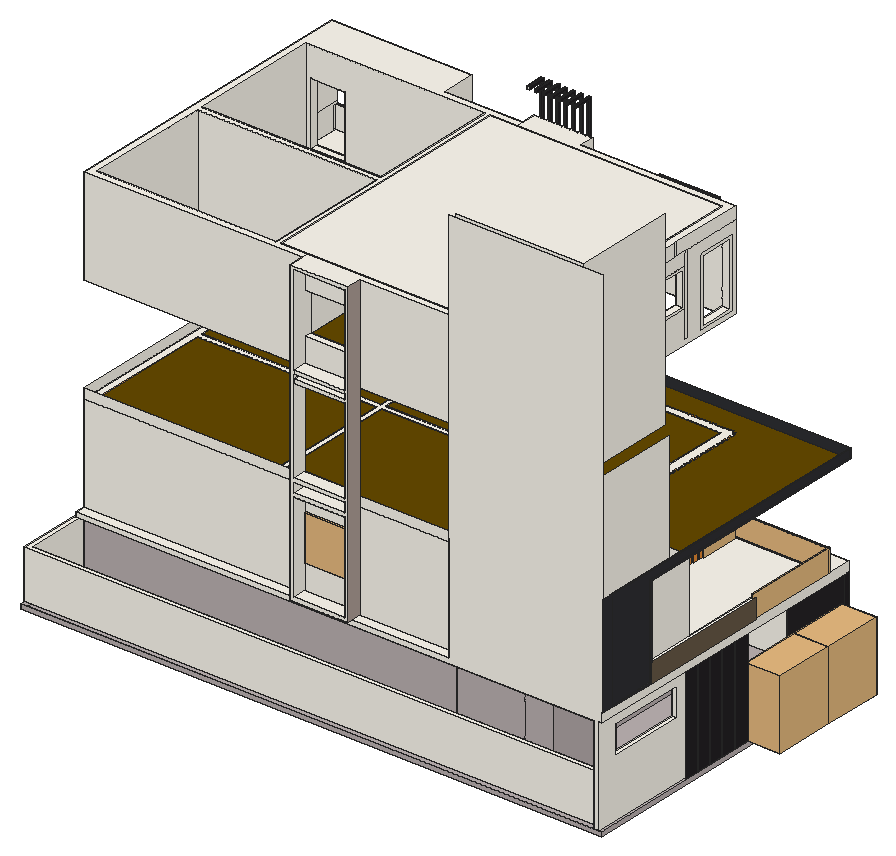
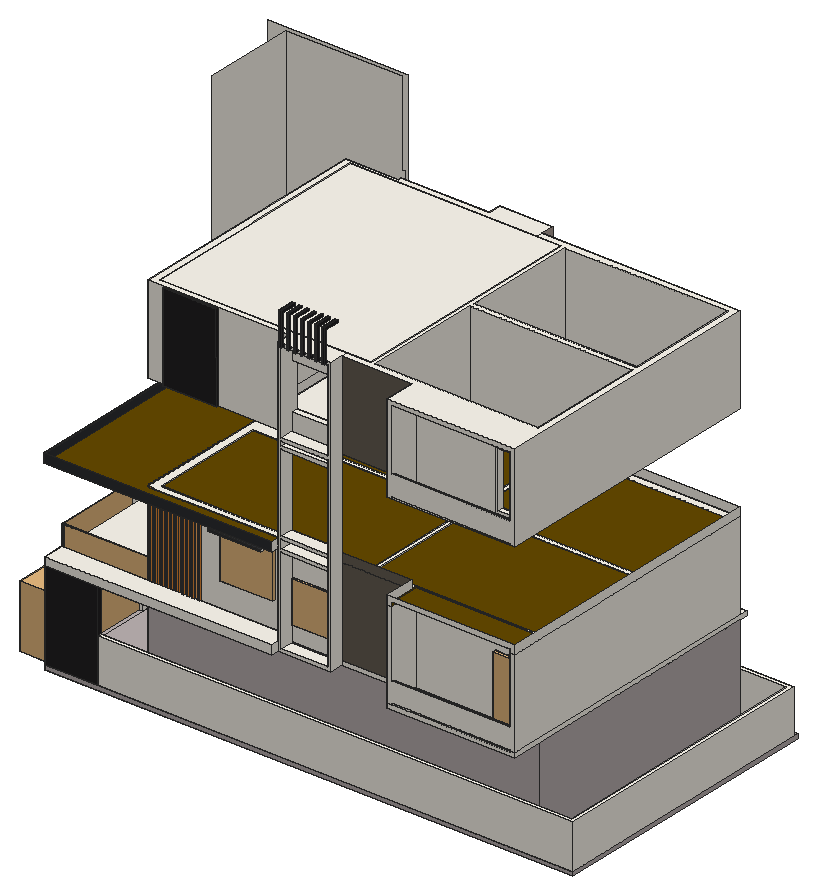
# SketchUp Ruby script. Lengths in inches.
U = 1.inch
M = Sketchup.active_model
def pt(a) = Geom::Point3d.new(a.map { |v| v * U })
def face(e, loops, mat)
  f = e.add_face(loops[0].map { |a| pt(a) })
  loops[1..].each { |l| e.add_face(l.map { |a| pt(a) }).erase! }
  f.material = f.back_material = mat if mat
  f
end
# faces: each face lists its corners as indices into pts; further lists are holes
def faces(e, pts, list, mat = nil) = list.each { |f| face(e, (f[0].is_a?(Array) ? f : [f]).map { |l| l.map { |i| pts[i] } }, mat) }
# xy, xz, yz: faces in a plane at the given z, y or x. An outline is a flat list of corners, or four numbers for a rectangle; further outlines are holes
def ring(l) = l.size == 4 ? [[l[0], l[1]], [l[2], l[1]], [l[2], l[3]], [l[0], l[3]]] : l.each_slice(2).to_a
def flat(e, list, mat, &to3) = list.each { |f| face(e, (f[0].is_a?(Array) ? f : [f]).map { |l| ring(l).map { |u, v| to3.(u, v) } }, mat) }
def xy(e, z, list, mat = nil) = flat(e, list, mat) { |x, y| [x, y, z] }
def xz(e, y, list, mat = nil) = flat(e, list, mat) { |x, z| [x, y, z] }
def yz(e, x, list, mat = nil) = flat(e, list, mat) { |y, z| [x, y, z] }
def lines(e, pts, list) = list.each { |a, b| e.add_line(pt(pts[a]), pt(pts[b])) }
# prism: a flat outline (further loops are holes) pulled along v
def prism(e, loops, v, mat = nil)
  f = face(e, loops, mat); d = Geom::Vector3d.new(v.map { |x| x * U })
  f.pushpull(f.normal.samedirection?(d) ? d.length : -d.length)
end
def box(e, o, s, mat = nil) = prism(e, [[o, [o[0] + s[0], o[1], o[2]], [o[0] + s[0], o[1] + s[1], o[2]], [o[0], o[1] + s[1], o[2]]]], [0, 0, s[2]], mat)
def at(x, y, z, deg = 0) = Geom::Transformation.translation(pt([x, y, z])) * Geom::Transformation.rotation(ORIGIN, Z_AXIS, deg.degrees)
def axes(o, x, y, z) = Geom::Transformation.new([*x, 0, *y, 0, *z, 0, *pt(o).to_a, 1])
def part(name) = M.definitions.add(name)
# library, detail: a bought-in or finely detailed component or shape, given as its bounding box
def library(name, o, s) = part(name).tap { |d| box(d.entities, o, s) }
def detail(e, o, s) = box(e.add_group.entities, o, s)
def put(e, d, t, mat = nil) = e.add_instance(d, t).tap { |i| i.material = mat if mat }
def group(e, t, mat = nil) = e.add_group.tap { |g| g.transformation = t; g.material = mat if mat }.entities
root = M.entities
M.materials.add("B04_Peach_Ember").color = [234, 141, 54]
M.materials.add("C01_Vanilla_Cream").color = [255, 251, 241]
M.materials.add("C03_Honey_Glow").color = [255, 178, 101]
M.materials.add("D08_Bronzed_Mustard").color = [102, 74, 0]
M.materials.add("Forest_Floor_01_1K").color = [106, 91, 72]
M.materials.add("Glass_Basic_1").color = [161, 173, 186]
M.materials["Glass_Basic_1"].alpha = 0.25
M.materials.add("Marble_07_1K").color = [36, 34, 36]
M.materials.add("Plaster_04_1K").color = [106, 98, 87]
M.materials.add("ThomThom - Buttons1").color = [48, 49, 53]
M.materials.add("ThomThom - Complexion1").color = [190, 180, 180]
M.materials.add("ThomThom - Hair1").color = [178, 163, 155]
c1 = library("porta+4",[0.2,-5.42,1.33],[46.55,4.72,83.21])
c2 = library("Ornamental gate leaf",[0,0,0],[161.42,42.43,280.3])
c3 = part("cong")
put(c3.entities,c2,axes([244.78,234.5625,0],[-1,0,0],[0,1,0],[0,0,1]))
put(c3.entities,c2,at(244.78,234.5625,0))
c4 = library("mesh-163",[-551.08,-704.17,-20.03],[1929.24,1401.85,86.96])
c5 = part("Group11")
put(c5.entities,c4,at(0,0,0))
c6 = library("Modern+Gate+1",[0,0,0],[118.11,1.97,78.74])
xy(root,0,[[0,6,720,389.16]],"ThomThom - Complexion1")
xy(root,6,[[711,6,717,138],[648,383.16,720,389.16]],"C01_Vanilla_Cream")
xy(root,6,[[0,6,9,389.16],[[9,6,711,389.16],[69,18,69,360,531,360,531,27,645,27,645,114,651,114,651,18]],[711,6,720,389.16],[78,27,300,183],[306,27,522,183],
  [78,189,300,351],[306,189,522,351]],"ThomThom - Complexion1")
xy(root,78,[[711,30,717,126]],"C01_Vanilla_Cream")
xy(root,114,[[711,30,717,126]],"C01_Vanilla_Cream")
xy(root,126,[[69,6,69,402,243,402,243,360,411,360,411,383.16,720,383.16,720,6,717,6,717,138,711,138,711,6],[411,383.16,648,389.16],[648,383.16,720,389.16]],"C01_Vanilla_Cream")
xy(root,126,[[531,18,651,18,651,114,645,114,645,27,531,27]],"ThomThom - Complexion1")
xy(root,132,[[69,6,531,6,531,190.4375,591.62,190.4375,591.62,348.27,531,348.27,531,360,243,360,243,402,69,402],[531,348.27,603,360]],"C01_Vanilla_Cream")
xy(root,138,[[537,12,693.41,12,693.41,144,718,144,718,241.67,720,241.67,720,357,603,357,603,348.27,591.62,348.27,591.62,190.4375,531,190.4375,531,24,537,24],[603,357,720,360],[411,360,720,389.16]],"C01_Vanilla_Cream")
xy(root,138,[[720,6,722,241.67]],"ThomThom - Buttons1")
xy(root,139,[[720,19,722,80]],"ThomThom - Buttons1")
xy(root,162,[[718,81,722,241.67]],"C01_Vanilla_Cream")
xy(root,252,[[537,12,603,24],[718,81,722,144]],"C01_Vanilla_Cream")
xy(root,252,[[69,18,69,402,75,402,75,360,237,360,237,402,243,402,243,360,411,360,411,389.16,722,389.16,722,144,603,144,603,24,531,24,531,18]],"D08_Bronzed_Mustard")
xy(root,253,[[720,80,722,144],[720,144,722,388.16]],"ThomThom - Buttons1")
xy(root,257.2,[[75,360,237,402]],"D08_Bronzed_Mustard")
xy(root,263,[[720,19,722,144],[720,144,722,388.16]],"ThomThom - Buttons1")
xz(root,6,[[711,6,717,6,717,126,720,126,720,138,722,138,722,624,531,624,531,132,69,132,69,126,711,126]],"C01_Vanilla_Cream")
xz(root,6,[[0,0,720,6]],"ThomThom - Complexion1")
xz(root,12,[[537,138,537,252,603,252,603,264,537,264,537,378,663.55,378,663.55,384,531,384,531,510,535,510,535,624,693.41,624,693.41,138]],"C01_Vanilla_Cream")
xz(root,18,[[69,252,531,264]],"C01_Vanilla_Cream")
xz(root,18,[[531,6,615,126],[615,6,651,126]],"ThomThom - Complexion1")
xz(root,19,[[720,139,722,263]],"ThomThom - Buttons1")
xz(root,24,[[531,138,537,252],[531,252,537,264],[537,252,603,264]],"C01_Vanilla_Cream")
xz(root,27,[[531,6,609,126],[609,6,642.82,126],[642.82,6,645,126]],"ThomThom - Complexion1")
xz(root,30,[[711,78,717,114]],"C01_Vanilla_Cream")
xz(root,80,[[720,139,722,253]],"ThomThom - Buttons1")
xz(root,81,[[718,162,722,252]],"C01_Vanilla_Cream")
xz(root,114,[[645,6,651,126]],"ThomThom - Complexion1")
xz(root,126,[[711,78,717,114]],"C01_Vanilla_Cream")
xz(root,144,[[693.41,138,718,252],[603,252,693.41,264]],"C01_Vanilla_Cream")
xz(root,190.4375,[[531,132,591.62,138]],"C01_Vanilla_Cream")
xz(root,241.67,[[718,138,722,162]],"C01_Vanilla_Cream")
xz(root,348.27,[[591.62,132,603,138]],"C01_Vanilla_Cream")
xz(root,360,[[243,126,411,132],[411,132,603,138]],"C01_Vanilla_Cream")
xz(root,360,[[75,252,237,257.2]],"D08_Bronzed_Mustard")
xz(root,360,[[243,252,411,264]],"Plaster_04_1K")
xz(root,360,[[[347.5,154.65,403.5,210.65],[351.5,158.65,399.5,206.65]]],"ThomThom - Complexion1")
xz(root,383.16,[[648,6,720,126]],"Marble_07_1K")
xz(root,388.16,[[720,253,722,263]],"ThomThom - Buttons1")
xz(root,389.16,[[411,126,720,138]],"C01_Vanilla_Cream")
xz(root,389.16,[[648,6,720,126]],"Marble_07_1K")
xz(root,389.16,[[411,252,722,264]],"ThomThom - Buttons1")
xz(root,389.16,[[0,0,720,6]],"ThomThom - Complexion1")
xz(root,402,[[69,126,243,132],[69,252,69,264,243,264,243,252,237,252,237,257.2,75,257.2,75,252]],"C01_Vanilla_Cream")
yz(root,0,[[6,0,389.16,6]],"ThomThom - Complexion1")
yz(root,69,[[6,126,402,132],[18,252,402,264]],"C01_Vanilla_Cream")
yz(root,75,[[360,252,402,257.2]],"D08_Bronzed_Mustard")
yz(root,237,[[360,252,402,257.2]],"D08_Bronzed_Mustard")
yz(root,243,[[360,126,402,132],[360,252,402,264]],"C01_Vanilla_Cream")
yz(root,411,[[360,126,389.16,138],[360,252,389.16,264]],"C01_Vanilla_Cream")
yz(root,531,[[6,132,6,252,24,252,24,138,190.4375,138,190.4375,132],[6,252,18,264],[18,252,24,264]],"C01_Vanilla_Cream")
yz(root,531,[[18,6,27,126]],"ThomThom - Complexion1")
yz(root,537,[[12,138,24,252]],"C01_Vanilla_Cream")
yz(root,591.62,[[190.4375,132,348.27,138]],"C01_Vanilla_Cream")
yz(root,603,[[348.27,132,360,138],[12,252,24,264],[24,252,144,264]],"C01_Vanilla_Cream")
yz(root,603,[[[240.57,42,288.57,90],[243.57,45,285.57,87]]],"ThomThom - Complexion1")
yz(root,645,[[27,6,114,126]],"ThomThom - Complexion1")
yz(root,648,[[383.16,66,389.16,126]],"Marble_07_1K")
yz(root,651,[[18,6,114,126]],"ThomThom - Complexion1")
yz(root,693.41,[[12,138,12,624,138,624,138,390,24,390,24,375,144,375,144,138]],"C01_Vanilla_Cream")
yz(root,711,[[[6,6,138,126],[30,78,126,114]]],"C01_Vanilla_Cream")
yz(root,717,[[[6,6,138,126],[30,78,126,114]]],"C01_Vanilla_Cream")
yz(root,718,[[144,138,241.67,162],[81,162,144,252]],"C01_Vanilla_Cream")
yz(root,720,[[6,126,389.16,138]],"C01_Vanilla_Cream")
yz(root,720,[[383.16,6,389.16,126]],"Marble_07_1K")
yz(root,720,[[19,139,80,139,80,253,388.16,253,388.16,263,19,263]],"ThomThom - Buttons1")
yz(root,720,[[6,0,389.16,6]],"ThomThom - Complexion1")
yz(root,722,[[81,138,241.67,162]],"Forest_Floor_01_1K")
yz(root,722,[[[6,138,81,138,81,252,389.16,252,389.16,264,6,264],[19,139,19,263,388.16,263,388.16,253,80,253,80,139]]],"ThomThom - Buttons1")
p = [[411,360,264],[411,360,126],[501.77,360,243],[498.77,360,243],[432.77,360,243],[429.77,360,243],
  [75,402,162],[75,399,162],[75,399,132],[603,348.27,138],[603,27,138],[531,360,138],
  [531,360,252]]
lines(root,p,[[0,1],[2,3],[3,4],[4,5],[6,7],[7,8],[9,10],[11,12]])
put(root,c1,axes([601.16,305.79,4.61],[0,1.03118,0],[-1,0,0],[0,0,1.01005]))
g1 = group(root,at(69,18,6),"ThomThom - Complexion1")
xy(g1,0,[[[0,0,0,342,534,342,534,9,462,9,462,0],[237,171,453,171,453,177,527.49,177,527.49,333,237,333],[9,171,231,333],[9,9,231,165],[237,9,453,165]]])
xy(g1,3,[[527.49,291,534,333]])
xy(g1,39,[[527.49,225.57,534,267.57]])
xy(g1,81,[[527.49,225.57,534,267.57],[527.49,291,534,333]])
xy(g1,120,[[[0,0,462,0,462,9,534,9,534,342,0,342],[237,171,237,333,527.49,333,527.49,177,453,177,453,171],[9,171,231,333],[9,9,231,165],[237,9,453,165]]])
xz(g1,0,[[0,0,462,120]])
xz(g1,9,[[9,0,231,120],[237,0,453,120],[462,0,534,120]])
xz(g1,165,[[9,0,231,120],[237,0,453,120]])
xz(g1,171,[[9,0,231,120],[237,0,453,120]])
xz(g1,177,[[453,0,527.49,120]])
xz(g1,225.57,[[527.49,39,534,81]])
xz(g1,267.57,[[527.49,39,534,81]])
xz(g1,291,[[527.49,3,534,81]])
xz(g1,333,[[9,0,231,120],[237,0,527.49,0,527.49,3,453,3,453,81,527.49,81,527.49,120,237,120],[453,3,534,81]])
xz(g1,342,[[0,0,534,120]])
yz(g1,0,[[0,0,342,120]])
yz(g1,9,[[9,0,165,120],[171,0,333,120]])
yz(g1,231,[[9,0,165,120],[171,0,333,120]])
yz(g1,237,[[9,0,165,120],[171,0,333,120]])
yz(g1,453,[[9,0,165,120],[171,0,177,120]])
yz(g1,462,[[0,0,9,120]])
yz(g1,527.49,[[[177,0,177,120,333,120,333,81,291,81,291,3,333,3,333,0],[225.57,39,267.57,81]]])
yz(g1,534,[[[9,0,288,0,288,84,336,84,336,0,342,0,342,120,9,120],[225.57,39,267.57,81]],[[288,0,336,84],[291,3,333,81]]])
g2 = group(root,at(711,138,6),"C01_Vanilla_Cream")
xy(g2,0,[[0,0,0,96,8,96,8,76.8,7,76.8,7,73.8,8,73.8,8,57.6,7,57.6,7,54.6,8,54.6,8,38.4,7,38.4,7,35.4,8,35.4,8,19.2,7,19.2,7,16.2,8,16.2,8,0]])
xy(g2,120,[[0,0,3,96],[3,0,8,0,8,16.2,7,16.2,7,19.2,8,19.2,8,35.4,7,35.4,7,38.4,8,38.4,8,54.6,7,54.6,7,57.6,8,57.6,8,73.8,7,73.8,7,76.8,8,76.8,8,96,3,96]])
xz(g2,0,[[0,0,8,120]])
xz(g2,16.2,[[7,0,8,120]])
xz(g2,19.2,[[7,0,8,120]])
xz(g2,35.4,[[7,0,8,120]])
xz(g2,38.4,[[7,0,8,120]])
xz(g2,54.6,[[7,0,8,120]])
xz(g2,57.6,[[7,0,8,120]])
xz(g2,73.8,[[7,0,8,120]])
xz(g2,76.8,[[7,0,8,120]])
xz(g2,96,[[0,0,8,120]])
yz(g2,0,[[0,0,96,120]])
yz(g2,7,[[16.2,0,19.2,120],[35.4,0,38.4,120],[54.6,0,57.6,120],[73.8,0,76.8,120]])
yz(g2,8,[[0,0,16.2,120],[19.2,0,35.4,120],[38.4,0,54.6,120],[57.6,0,73.8,120],[76.8,0,96,120]],"Marble_07_1K")
g3 = group(root,at(648,383.16,6),"C01_Vanilla_Cream")
prism(g3,[[[0,6,0],[0,0,0],[-642,0,0],[-642,-365.16,0],[63,-365.16,0],[63,-371.16,0],[-648,-371.16,0],[-648,6,0]]],[0,0,60])
put(root,c3,axes([993.24,195.48,6],[0,0.46204,0],[-1,0,0],[0,0,0.3061]))
put(root,c5,axes([603.79,254.28,66.08],[0,0.02488,0],[0,0,0.0342],[0.03937,0,0]))
g4 = group(root,at(69,18,384),"C01_Vanilla_Cream")
xy(g4,-258,[[270,342,274,360],[274,342,342,360]])
xy(g4,-254,[[274,342,338,360]])
xy(g4,-252,[[270,-18,274,0],[274,-18,342,0]])
xy(g4,-248,[[274,-18,338,0]])
xy(g4,-136,[[274,-18,338,0]])
xy(g4,-135.99,[[274,342,338,360]])
xy(g4,-132,[[274,-18,338,0]])
xy(g4,-131.99,[[274,342,338,360]])
xy(g4,-120,[[274,-18,338,0],[274,342,338,360]])
xy(g4,-116,[[274,-18,338,0],[274,342,338,360]])
xy(g4,-10,[[274,-18,338,0],[274,342,338,360]])
xy(g4,-6,[[274,-18,338,0],[274,342,338,360]])
xy(g4,0,[[[274,-18,274,0,0,0,0,384,6,384,6,342,168,342,168,384,174,384,174,342,274,342,274,360,338,360,338,342,534,342,534,4.78,462,4.78,462,0,338,0,338,-18],[237,9,524.52,333],[9,171,231,333],[9,9,231,165]],[6,342,168,384]])
xy(g4,2,[[6,342,168,381],[6,381,168,384]])
xy(g4,4,[[274,-18,338,0]])
xy(g4,4,[[274,342,338,360]],"C01_Vanilla_Cream")
xy(g4,5,[[15,333,57,342]])
xy(g4,9,[[524.52,291,534,333]])
xy(g4,28,[[274,333,338,342]])
xy(g4,29.9375,[[6,381,168,384]])
xy(g4,33.78,[[274,0,338,9]])
xy(g4,42.51,[[524.52,218.59,534,225.89],[524.52,225.89,534,228.89],[524.52,228.89,534,260.59]],"C01_Vanilla_Cream")
xy(g4,83,[[15,333,57,342]])
xy(g4,84.51,[[524.52,218.59,534,225.89],[524.52,225.89,534,228.89],[524.52,228.89,534,260.59]],"C01_Vanilla_Cream")
xy(g4,85.33,[[274,0,338,9]])
xy(g4,87,[[524.52,291,534,333]])
xy(g4,90.72,[[274,333,338,342]])
xy(g4,114,[[6,342,168,384]])
xy(g4,116,[[274,-18,338,0],[274,342,338,360]])
xy(g4,117,[[275.47,360,278.47,364],[285.24,360,288.24,364],[295.02,360,298.02,364],[304.79,360,307.79,364],[314.57,360,317.57,364],
  [324.34,360,327.34,364],[334.11,360,337.11,364]],"Marble_07_1K")
xy(g4,120,[[[0,0,270,0,270,9,237,9,237,333,270,333,270,342,174,342,174,384,0,384],[9,171,231,333],[9,9,231,165]],[237,9,524.52,333]])
xy(g4,120,[[270,-18,342,-18,342,0,462,0,462,4.78,534,4.78,534,342,342,342,342,360,337.11,360,337.11,362,334.11,362,334.11,360,327.34,360,327.34,362,324.34,362,324.34,360,317.57,360,317.57,362,314.57,362,314.57,360,307.79,360,307.79,362,304.79,362,304.79,360,298.02,360,298.02,362,295.02,362,295.02,360,288.24,360,288.24,362,285.24,362,285.24,360,278.47,360,278.47,362,275.47,362,275.47,360,270,360,270,333,524.52,333,524.52,9,270,9]],"C01_Vanilla_Cream")
xy(g4,159,[[275.47,342,278.47,362],[285.24,342,288.24,362],[295.02,342,298.02,362],[304.79,342,307.79,362],[314.57,342,317.57,362],
  [324.34,342,327.34,362],[334.11,342,337.11,362]],"Marble_07_1K")
xy(g4,162,[[275.47,342,278.47,364],[285.24,342,288.24,364],[295.02,342,298.02,364],[304.79,342,307.79,364],[314.57,342,317.57,364],
  [324.34,342,327.34,364],[334.11,342,337.11,364]],"Marble_07_1K")
xz(g4,-18,[[[270,-252,342,120],[274,-6,338,116],[274,-248,338,-136],[274,-116,338,-10],[274,-132,338,-120]],[274,0,338,4]])
xz(g4,0,[[270,-252,274,0],[274,-252,274,-248,338,-248,338,-136,274,-136,274,-132,338,-132,338,-120,274,-120,274,-116,338,-116,338,-10,274,-10,274,-6,338,-6,338,0,342,0,342,-252],[0,0,270,120],[342,0,462,120],[274,4,338,33.78],
  [274,85.33,338,116]])
xz(g4,4.78,[[462,0,534,120]])
xz(g4,9,[[9,0,231,120],[[237,0,524.52,120],[274,33.78,338,85.33]]])
xz(g4,165,[[9,0,231,120]])
xz(g4,171,[[9,0,231,120]])
xz(g4,218.59,[[524.52,42.51,534,84.51]],"C01_Vanilla_Cream")
xz(g4,260.59,[[524.52,42.51,534,84.51]],"C01_Vanilla_Cream")
xz(g4,291,[[524.52,9,534,87]])
xz(g4,333,[[[9,0,231,120],[15,5,57,83]],[[237,0,524.52,120],[274,28,338,90.72]],[524.52,9,534,87],[6,28.09,9,90.72]])
xz(g4,342,[[270,-258,274,0],[274,-258,342,-258,342,0,338,0,338,-6,274,-6,274,-10,338,-10,338,-116,274,-116,274,-120,338,-120,338,-131.99,274,-131.99,274,-135.99,338,-135.99,338,-254,274,-254],[6,0,168,2],[342,0,534,120],[[12,2,60,86],[15,5,57,83]]])
xz(g4,342,[[6,2,6,114,168,114,168,2,60,2,60,86,12,86,12,2],[274,4,338,28],[274,90.72,338,116],[275.47,159,278.47,162],[285.24,159,288.24,162],
  [295.02,159,298.02,162],[304.79,159,307.79,162],[314.57,159,317.57,162],[324.34,159,327.34,162],[334.11,159,337.11,162]],"C01_Vanilla_Cream")
xz(g4,342,[[174,0,270,120]],"Plaster_04_1K")
xz(g4,360,[[[270,-258,270,120,275.47,120,275.47,117,278.47,117,278.47,120,285.24,120,285.24,117,288.24,117,288.24,120,295.02,120,295.02,117,298.02,117,298.02,120,304.79,120,304.79,117,307.79,117,307.79,120,314.57,120,314.57,117,317.57,117,317.57,120,324.34,120,324.34,117,327.34,117,327.34,120,334.11,120,334.11,117,337.11,117,337.11,120,342,120,342,-258],[274,-254,338,-135.99],[274,4,338,116],[274,-116,338,-10],[274,-131.99,338,-120],[274,-6,338,0]]],"C01_Vanilla_Cream")
xz(g4,362,[[275.47,120,278.47,159],[285.24,120,288.24,159],[295.02,120,298.02,159],[304.79,120,307.79,159],[314.57,120,317.57,159],
  [324.34,120,327.34,159],[334.11,120,337.11,159]],"Marble_07_1K")
xz(g4,364,[[275.47,117,278.47,162],[285.24,117,288.24,162],[295.02,117,298.02,162],[304.79,117,307.79,162],[314.57,117,317.57,162],
  [324.34,117,327.34,162],[334.11,117,337.11,162]],"Marble_07_1K")
xz(g4,381,[[6,2,168,29.9375]])
xz(g4,384,[[6,0,168,2]])
xz(g4,384,[[[0,0,0,120,174,120,174,0,168,0,168,2,6,2,6,0],[6,29.9375,168,114]]],"C01_Vanilla_Cream")
yz(g4,0,[[0,0,384,120]])
yz(g4,6,[[342,0,384,2],[378,2,381,29.9375]])
yz(g4,6,[[342,2,378,2,378,29.9375,384,29.9375,384,32,342,32],[342,32,384,114]],"C01_Vanilla_Cream")
yz(g4,9,[[9,0,165,120],[171,0,333,120]])
yz(g4,15,[[333,5,342,83]],"C01_Vanilla_Cream")
yz(g4,57,[[333,5,342,83]])
yz(g4,168,[[342,0,384,2]])
yz(g4,168,[[342,2,342,114,384,114,384,29.9375,381,29.9375,381,2]],"C01_Vanilla_Cream")
yz(g4,174,[[342,0,384,120]],"C01_Vanilla_Cream")
yz(g4,231,[[9,0,165,120],[171,0,333,120]])
yz(g4,237,[[9,0,171,120],[171,0,333,120]])
yz(g4,270,[[342,-258,360,120]],"C01_Vanilla_Cream")
yz(g4,270,[[-18,-252,0,120]],"ThomThom - Hair1")
yz(g4,274,[[342,-254,360,-135.99],[-18,-248,0,-136],[342,-135.99,360,-131.99],[-18,-132,0,-120],[342,-131.99,360,-120],
  [342,-120,360,-116],[-18,-116,0,-10],[342,-116,360,-10],[-18,-10,0,-6],[342,-10,360,-6],
  [-18,-6,0,0],[342,-6,360,0],[-18,4,0,4,0,33.78,9,33.78,9,85.33,0,85.33,0,116,-18,116]])
yz(g4,274,[[342,4,360,4,360,116,342,116,342,90.72,333,90.72,333,28,342,28]],"C01_Vanilla_Cream")
yz(g4,275.47,[[360,117,360,120,362,120,362,159,342,159,342,162,364,162,364,117]],"Marble_07_1K")
yz(g4,278.47,[[360,117,364,117,364,162,342,162,342,159,362,159,362,120,360,120]],"Marble_07_1K")
yz(g4,285.24,[[360,117,360,120,362,120,362,159,342,159,342,162,364,162,364,117]],"Marble_07_1K")
yz(g4,288.24,[[360,117,364,117,364,162,342,162,342,159,362,159,362,120,360,120]],"Marble_07_1K")
yz(g4,295.02,[[360,117,360,120,362,120,362,159,342,159,342,162,364,162,364,117]],"Marble_07_1K")
yz(g4,298.02,[[360,117,364,117,364,162,342,162,342,159,362,159,362,120,360,120]],"Marble_07_1K")
yz(g4,304.79,[[360,117,360,120,362,120,362,159,342,159,342,162,364,162,364,117]],"Marble_07_1K")
yz(g4,307.79,[[360,117,364,117,364,162,342,162,342,159,362,159,362,120,360,120]],"Marble_07_1K")
yz(g4,314.57,[[360,117,360,120,362,120,362,159,342,159,342,162,364,162,364,117]],"Marble_07_1K")
yz(g4,317.57,[[360,117,364,117,364,162,342,162,342,159,362,159,362,120,360,120]],"Marble_07_1K")
yz(g4,324.34,[[360,117,360,120,362,120,362,159,342,159,342,162,364,162,364,117]],"Marble_07_1K")
yz(g4,327.34,[[360,117,364,117,364,162,342,162,342,159,362,159,362,120,360,120]],"Marble_07_1K")
yz(g4,334.11,[[360,117,360,120,362,120,362,159,342,159,342,162,364,162,364,117]],"Marble_07_1K")
yz(g4,337.11,[[360,117,364,117,364,162,342,162,342,159,362,159,362,120,360,120]],"Marble_07_1K")
yz(g4,338,[[342,-254,360,-135.99],[-18,-248,0,-136],[-18,-132,0,-120],[342,-131.99,360,-120],[-18,-116,0,-10],
  [342,-116,360,-10],[-18,-6,0,0],[342,-6,360,0],[-18,4,-18,116,0,116,0,85.33,9,85.33,9,33.78,0,33.78,0,4]])
yz(g4,338,[[342,4,342,28,333,28,333,90.72,342,90.72,342,116,360,116,360,4]],"C01_Vanilla_Cream")
yz(g4,342,[[342,-258,360,120]],"C01_Vanilla_Cream")
yz(g4,342,[[-18,-252,0,120]],"ThomThom - Hair1")
yz(g4,438,[[344,-0.02,342,0,343.1875,120,345.1875,119.98]],"Marble_07_1K")
yz(g4,462,[[0,0,4.78,120]])
yz(g4,511.45,[[344,-0.02,345.1875,119.98,343.1875,120,342,0]],"Marble_07_1K")
yz(g4,524.52,[[9,0,171,120],[171,0,177,120],[[177,0,177,120,333,120,333,87,291,87,291,9,333,9,333,0],[218.59,42.51,260.59,84.51]]])
yz(g4,534,[[288,6,304.3,6,304.3,9,291,9,291,87,333,87,333,9,304.3,9,304.3,6,336,6,336,90,288,90]])
yz(g4,534,[[[4.78,0,342,0,342,103.96,266.59,103.96,266.59,6,263.59,6,263.59,39.51,228.89,39.51,228.89,6,225.89,6,225.89,39.51,215.59,39.51,215.59,87.51,225.89,87.51,225.89,103.96,191.18,103.96,191.18,6,188.18,6,188.18,103.96,153.48,103.96,153.48,6,150.48,6,150.48,103.96,115.18,103.96,115.18,6,112.18,6,112.18,103.96,75.25,103.96,75.25,6,72.25,6,72.25,103.96,4.78,103.96],[288,6,336,90]],[72.25,6,75.25,103.96],[112.18,6,115.18,103.96],[150.48,6,153.48,103.96],[188.18,6,191.18,103.96],
  [225.89,6,228.89,39.51],[263.59,6,266.59,103.96],[[215.59,39.51,263.59,87.51],[218.59,42.51,260.59,84.51]],[225.89,87.51,228.89,103.96],[228.89,87.51,263.59,103.96],
  [4.78,103.96,93.72,120],[93.72,103.96,96.77,120],[96.77,103.96,133.125,120],[133.125,103.96,136.125,120],[136.125,103.96,170.83,120],
  [170.83,103.96,173.83,120],[173.83,103.96,208.53,120],[208.53,103.96,211.53,120],[211.53,103.96,246.24,120],[246.24,103.96,249.24,120],
  [249.24,103.96,342,120]],"C01_Vanilla_Cream")
p = [[511.45,342,0],[511.45,343.1875,120],[438,343.1875,120],[438,342,0],[438,344,-0.02],[511.45,344,-0.02],
  [511.45,345.1875,119.98],[438,345.1875,119.98],[274,342,90.72],[270,342,90.72],[174,342,90.72],[168,342,90.72],
  [534,115.77,0],[534,115.77,6],[278.47,362,159],[285.24,362,159],[288.24,362,159],[295.02,362,159],
  [298.02,362,159],[304.79,362,159],[307.79,362,159],[314.57,362,159],[317.57,362,159],[324.34,362,159],
  [327.34,362,159],[334.11,362,159]]
faces(g4,p,[[0,1,2,3],[0,3,4,5],[6,5,4,7],[2,1,6,7]],"Marble_07_1K")
lines(g4,p,[[8,9],[10,11],[12,13],[14,15],[16,17],[18,19],[20,21],[22,23],[24,25]])
g5 = group(root,at(69,18,132),"C01_Vanilla_Cream")
xy(g5,0,[[6,342,168,384]])
xy(g5,0,[[[0,0,0,384,6,384,6,342,168,342,168,384,174,384,174,342,534,342,534,9,462,9,462,0],[237,171,453,171,453,177,522.62,177,522.62,333,237,333],[9,171,231,333],[9,9,231,165],[237,9,453,165]]],"C03_Honey_Glow")
xy(g5,2,[[6,342,168,381],[6,381,168,384]])
xy(g5,5,[[15,333,57,342]])
xy(g5,6,[[534,336,536,337.8]],"B04_Peach_Ember")
xy(g5,6,[[534,216,536,220.2],[534,224.4,536,228.6],[534,232.8,536,237],[534,241.2,536,245.4],[534,249.6,536,253.8],
  [534,258,536,262.2],[534,266.4,536,270.6],[534,274.8,536,279],[534,283.2,536,287.4],[533.97,337.8,534,339.9],
  [462,342,465.6,343],[469.2,342,472.8,343],[476.4,342,480,343],[483.6,342,487.2,343],[490.8,342,494.4,343],
  [498,342,501.6,343],[505.2,342,508.8,343],[512.4,342,516,343],[519.6,342,523.2,343],[526.8,342,530.4,343]],"C03_Honey_Glow")
xy(g5,9,[[522.62,291,534,333]])
xy(g5,26.65,[[282.5,333,330.5,342]])
xy(g5,29.53,[[6,381,168,384]])
xy(g5,40.93,[[279.92,0,327.92,9]])
xy(g5,45,[[363.77,333,429.77,342]])
xy(g5,74.65,[[282.5,333,330.5,342]])
xy(g5,83,[[15,333,57,342]])
xy(g5,87,[[522.62,291,534,333]])
xy(g5,88.93,[[279.92,0,327.92,9]])
xy(g5,90,[[534,333.6,536,336]],"B04_Peach_Ember")
xy(g5,90,[[534,291.6,536,295.8],[534,300,536,304.2],[534,308.4,536,312.6],[534,316.8,536,321],[534,325.2,536,329.4]],"C03_Honey_Glow")
xy(g5,111,[[363.77,333,429.77,366],[360.77,342,363.77,366],[429.77,342,432.77,366]],"ThomThom - Buttons1")
xy(g5,114,[[360.77,342,432.77,366]],"ThomThom - Buttons1")
xy(g5,120,[[[0,0,462,0,462,9,534,9,534,216,536,216,536,220.2,534,220.2,534,224.4,536,224.4,536,228.6,534,228.6,534,232.8,536,232.8,536,237,534,237,534,241.2,536,241.2,536,245.4,534,245.4,534,249.6,536,249.6,536,253.8,534,253.8,534,258,536,258,536,262.2,534,262.2,534,266.4,536,266.4,536,270.6,534,270.6,534,274.8,536,274.8,536,279,534,279,534,283.2,536,283.2,536,287.4,534,287.4,534,291.6,536,291.6,536,295.8,534,295.8,534,300,536,300,536,304.2,534,304.2,534,308.4,536,308.4,536,312.6,534,312.6,534,316.8,536,316.8,536,321,534,321,534,325.2,536,325.2,536,329.4,534,329.4,534,333.6,536,333.6,536,337.8,533.97,337.8,533.97,339.9,534,339.9,534,342,530.4,342,530.4,343,526.8,343,526.8,342,523.2,342,523.2,343,519.6,343,519.6,342,516,342,516,343,512.4,343,512.4,342,508.8,342,508.8,343,505.2,343,505.2,342,501.6,342,501.6,343,498,343,498,342,494.4,342,494.4,343,490.8,343,490.8,342,487.2,342,487.2,343,483.6,343,483.6,342,480,342,480,343,476.4,343,476.4,342,472.8,342,472.8,343,469.2,343,469.2,342,465.6,342,465.6,343,462,343,462,342,174,342,174,384,168,384,168,342,6,342,6,384,0,384],[237,171,237,333,522.62,333,522.62,177,453,177,453,171],[9,171,231,333],[9,9,231,165],[237,9,453,165]]])
xz(g5,0,[[[0,0,462,120],[276.92,37.93,330.92,91.93]],[[276.92,37.93,330.92,91.93],[279.92,40.93,327.92,88.93]]])
xz(g5,9,[[9,0,231,120],[[237,0,453,120],[279.92,40.93,327.92,88.93]],[462,0,534,120]],"C03_Honey_Glow")
xz(g5,165,[[237,0,453,120]])
xz(g5,165,[[9,0,231,120]],"C03_Honey_Glow")
xz(g5,171,[[9,0,231,120],[237,0,453,120]])
xz(g5,177,[[453,0,522.62,120]])
xz(g5,216,[[534,6,536,120]],"B04_Peach_Ember")
xz(g5,220.2,[[534,6,536,120]],"B04_Peach_Ember")
xz(g5,224.4,[[534,6,536,120]],"B04_Peach_Ember")
xz(g5,228.6,[[534,6,536,120]],"B04_Peach_Ember")
xz(g5,232.8,[[534,6,536,120]],"B04_Peach_Ember")
xz(g5,237,[[534,6,536,120]],"B04_Peach_Ember")
xz(g5,241.2,[[534,6,536,120]],"B04_Peach_Ember")
xz(g5,245.4,[[534,6,536,120]],"B04_Peach_Ember")
xz(g5,249.6,[[534,6,536,120]],"B04_Peach_Ember")
xz(g5,253.8,[[534,6,536,120]],"B04_Peach_Ember")
xz(g5,258,[[534,6,536,120]],"B04_Peach_Ember")
xz(g5,262.2,[[534,6,536,120]],"B04_Peach_Ember")
xz(g5,266.4,[[534,6,536,120]],"B04_Peach_Ember")
xz(g5,270.6,[[534,6,536,120]],"B04_Peach_Ember")
xz(g5,274.8,[[534,6,536,120]],"B04_Peach_Ember")
xz(g5,279,[[534,6,536,120]],"B04_Peach_Ember")
xz(g5,283.2,[[534,6,536,120]],"B04_Peach_Ember")
xz(g5,287.4,[[534,6,536,120]],"B04_Peach_Ember")
xz(g5,291,[[522.62,9,534,87]])
xz(g5,291.6,[[534,90,536,120]],"B04_Peach_Ember")
xz(g5,295.8,[[534,90,536,120]],"B04_Peach_Ember")
xz(g5,300,[[534,90,536,120]],"B04_Peach_Ember")
xz(g5,304.2,[[534,90,536,120]],"B04_Peach_Ember")
xz(g5,308.4,[[534,90,536,120]],"B04_Peach_Ember")
xz(g5,312.6,[[534,90,536,120]],"B04_Peach_Ember")
xz(g5,316.8,[[534,90,536,120]],"B04_Peach_Ember")
xz(g5,321,[[534,90,536,120]],"B04_Peach_Ember")
xz(g5,325.2,[[534,90,536,120]],"B04_Peach_Ember")
xz(g5,329.4,[[534,90,536,120]],"B04_Peach_Ember")
xz(g5,333,[[[9,0,231,120],[15,5,57,83]],[[237,0,522.62,0,522.62,9,534,9,534,87,522.62,87,522.62,120,237,120],[363.77,45,429.77,111],[282.5,26.65,330.5,74.65]]])
xz(g5,333.6,[[534,90,536,120]],"B04_Peach_Ember")
xz(g5,336,[[534,6,536,90]],"B04_Peach_Ember")
xz(g5,337.8,[[533.97,6,536,120]],"C03_Honey_Glow")
xz(g5,339.9,[[533.97,6,534,120]],"C03_Honey_Glow")
xz(g5,342,[[6,0,168,2],[[270,0,270,120,462,120,462,6,534,6,534,0],[360.77,42,432.77,114],[282.5,26.65,330.5,74.65]],[[12,2,60,86],[15,5,57,83]],[360.77,42,360.77,111,363.77,111,363.77,45,429.77,45,429.77,111,432.77,111,432.77,42]])
xz(g5,342,[[6,2,6,120,168,120,168,2,60,2,60,86,12,86,12,2]],"C01_Vanilla_Cream")
xz(g5,342,[[465.6,6,469.2,120],[472.8,6,476.4,120],[480,6,483.6,120],[487.2,6,490.8,120],[494.4,6,498,120],
  [501.6,6,505.2,120],[508.8,6,512.4,120],[516,6,519.6,120],[523.2,6,526.8,120],[530.4,6,534,120]],"C03_Honey_Glow")
xz(g5,342,[[174,0,270,120]],"Plaster_04_1K")
xz(g5,343,[[462,6,465.6,120],[469.2,6,472.8,120],[476.4,6,480,120],[483.6,6,487.2,120],[490.8,6,494.4,120],
  [498,6,501.6,120],[505.2,6,508.8,120],[512.4,6,516,120],[519.6,6,523.2,120],[526.8,6,530.4,120]],"B04_Peach_Ember")
xz(g5,366,[[360.77,111,432.77,114]],"ThomThom - Buttons1")
xz(g5,381,[[6,2,168,29.53]])
xz(g5,384,[[6,0,168,2]])
xz(g5,384,[[0,0,0,120,6,120,6,29.53,168,29.53,168,120,174,120,174,0,168,0,168,2,6,2,6,0]],"C01_Vanilla_Cream")
yz(g5,0,[[0,0,384,120]])
yz(g5,6,[[342,0,381,2],[381,0,384,2],[342,2,381,2,381,29.53,384,29.53,384,120,342,120]])
yz(g5,9,[[171,0,333,120]])
yz(g5,9,[[9,0,165,120]],"C03_Honey_Glow")
yz(g5,15,[[333,5,342,83]])
yz(g5,57,[[333,5,342,83]])
yz(g5,168,[[342,0,384,2],[342,2,342,120,384,120,384,29.53,381,29.53,381,2]])
yz(g5,174,[[342,0,384,120]])
yz(g5,231,[[171,0,333,120]])
yz(g5,231,[[9,0,165,120]],"C03_Honey_Glow")
yz(g5,237,[[9,0,165,120],[171,0,333,120]])
yz(g5,279.92,[[0,40.93,9,88.93]])
yz(g5,282.5,[[333,26.65,342,74.65]])
yz(g5,327.92,[[0,40.93,9,88.93]])
yz(g5,330.5,[[333,26.65,342,74.65]])
yz(g5,360.77,[[342,111,366,114]])
yz(g5,363.77,[[333,45,342,111]])
yz(g5,429.77,[[333,45,342,111]])
yz(g5,432.77,[[342,111,366,114]],"ThomThom - Buttons1")
yz(g5,453,[[9,0,165,120]])
yz(g5,453,[[171,0,177,120]],"C03_Honey_Glow")
yz(g5,462,[[342,6,343,120]],"B04_Peach_Ember")
yz(g5,462,[[0,0,9,120]],"C03_Honey_Glow")
yz(g5,465.6,[[342,6,343,120]],"B04_Peach_Ember")
yz(g5,469.2,[[342,6,343,120]],"B04_Peach_Ember")
yz(g5,472.8,[[342,6,343,120]],"B04_Peach_Ember")
yz(g5,476.4,[[342,6,343,120]],"B04_Peach_Ember")
yz(g5,480,[[342,6,343,120]],"B04_Peach_Ember")
yz(g5,483.6,[[342,6,343,120]],"B04_Peach_Ember")
yz(g5,487.2,[[342,6,343,120]],"B04_Peach_Ember")
yz(g5,490.8,[[342,6,343,120]],"B04_Peach_Ember")
yz(g5,494.4,[[342,6,343,120]],"B04_Peach_Ember")
yz(g5,498,[[342,6,343,120]],"B04_Peach_Ember")
yz(g5,501.6,[[342,6,343,120]],"B04_Peach_Ember")
yz(g5,505.2,[[342,6,343,120]],"B04_Peach_Ember")
yz(g5,508.8,[[342,6,343,120]],"B04_Peach_Ember")
yz(g5,512.4,[[342,6,343,120]],"B04_Peach_Ember")
yz(g5,516,[[342,6,343,120]],"B04_Peach_Ember")
yz(g5,519.6,[[342,6,343,120]],"B04_Peach_Ember")
yz(g5,522.62,[[177,0,177,120,333,120,333,87,291,87,291,9,333,9,333,0]])
yz(g5,523.2,[[342,6,343,120]],"B04_Peach_Ember")
yz(g5,526.8,[[342,6,343,120]],"B04_Peach_Ember")
yz(g5,530.4,[[342,6,343,120]],"B04_Peach_Ember")
yz(g5,533.97,[[337.8,6,339.9,120]],"C03_Honey_Glow")
yz(g5,534,[[339.9,6,342,120]],"B04_Peach_Ember")
yz(g5,534,[[220.2,6,224.4,120],[228.6,6,232.8,120],[237,6,241.2,120],[245.4,6,249.6,120],[253.8,6,258,120],
  [262.2,6,266.4,120],[270.6,6,274.8,120],[279,6,283.2,120],[287.4,6,288,6,288,90,291.6,90,291.6,120,287.4,120],[[288,6,336,90],[291,9,333,87]],
  [295.8,90,300,120],[304.2,90,308.4,120],[312.6,90,316.8,120],[321,90,325.2,120],[329.4,90,333.6,120]],"C03_Honey_Glow")
yz(g5,534,[[146.76,40.58,188.76,82.58]],"Glass_Basic_1")
yz(g5,534,[[[9,0,342,0,342,6,216,6,216,120,9,120],[143.76,37.58,191.76,85.58]],[[143.76,37.58,191.76,85.58],[146.76,40.58,188.76,82.58]]],"ThomThom - Hair1")
yz(g5,536,[[216,6,220.2,120],[224.4,6,228.6,120],[232.8,6,237,120],[241.2,6,245.4,120],[249.6,6,253.8,120],
  [258,6,262.2,120],[266.4,6,270.6,120],[274.8,6,279,120],[283.2,6,287.4,120],[336,6,337.8,6,337.8,120,333.6,120,333.6,90,336,90],
  [291.6,90,295.8,120],[300,90,304.2,120],[308.4,90,312.6,120],[316.8,90,321,120],[325.2,90,329.4,120]],"B04_Peach_Ember")
p = [[462,341.81,6],[462,342,120],[453,333,9],[522.62,333,9],[270,342,132],[270,342,120],
  [624.41,126,6],[534,126,6]]
lines(g5,p,[[0,1],[2,3],[4,5],[6,7]])
put(root,c1,axes([129.21,359.3,132.66],[-1.03118,0,0],[0,-1,0],[0,0,1.00971]))
put(root,c6,axes([603,358.03,138],[0.99087,0,0],[0,1,0],[0,0,0.34577]))
put(root,c6,axes([720.02,240.94,138],[0,1.008,0],[-1,0,0],[0,0,0.34765]))
put(root,c1,axes([601.16,305.79,136.81],[0,1.03118,0],[-1,0,0],[0,0,1.01005]))
put(root,c5,axes([387.26,360.79,182.73],[-0.02948,0,0],[0,0,0.03987],[0,0.03937,0]))
put(root,c5,axes([385.65,15.37,196.52],[-0.02883,0,0],[0,0,0.03929],[0,0.03937,0]))
put(root,c5,axes([603.77,175.47,193.66],[0,0.02488,0],[0,0,0.0342],[0.03937,0,0]))
put(root,c5,axes([481.21,360.79,208.66],[-0.03732,0,0],[0,0,0.04922],[0,0.03937,0]))
